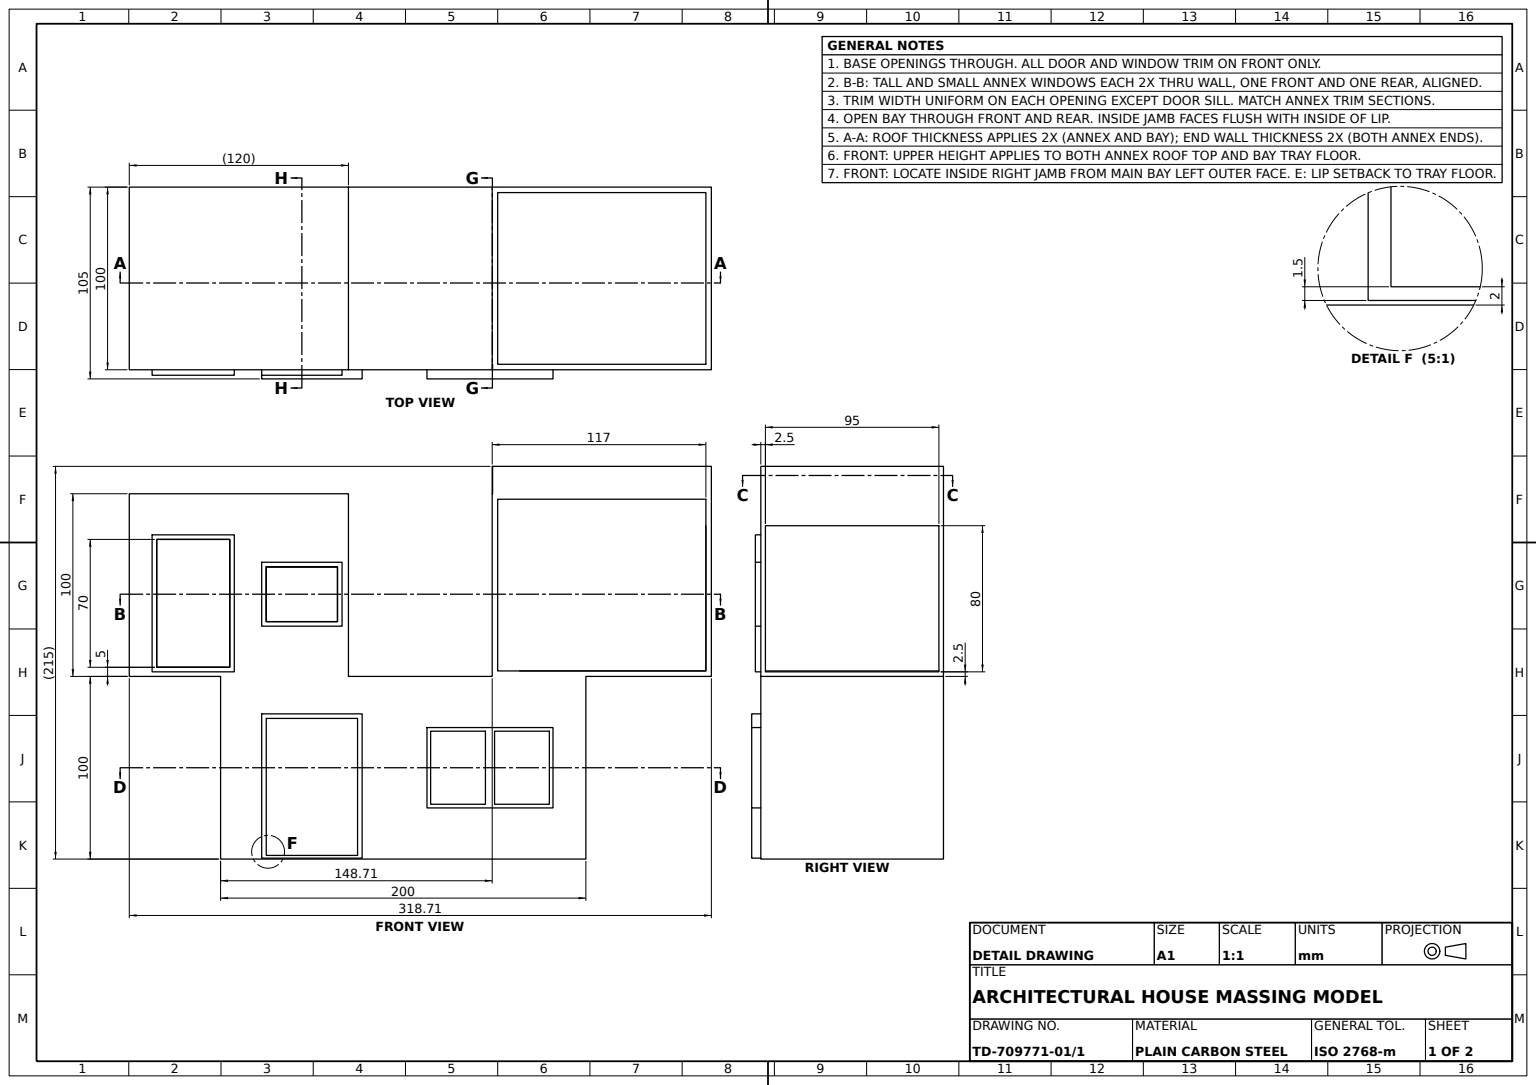
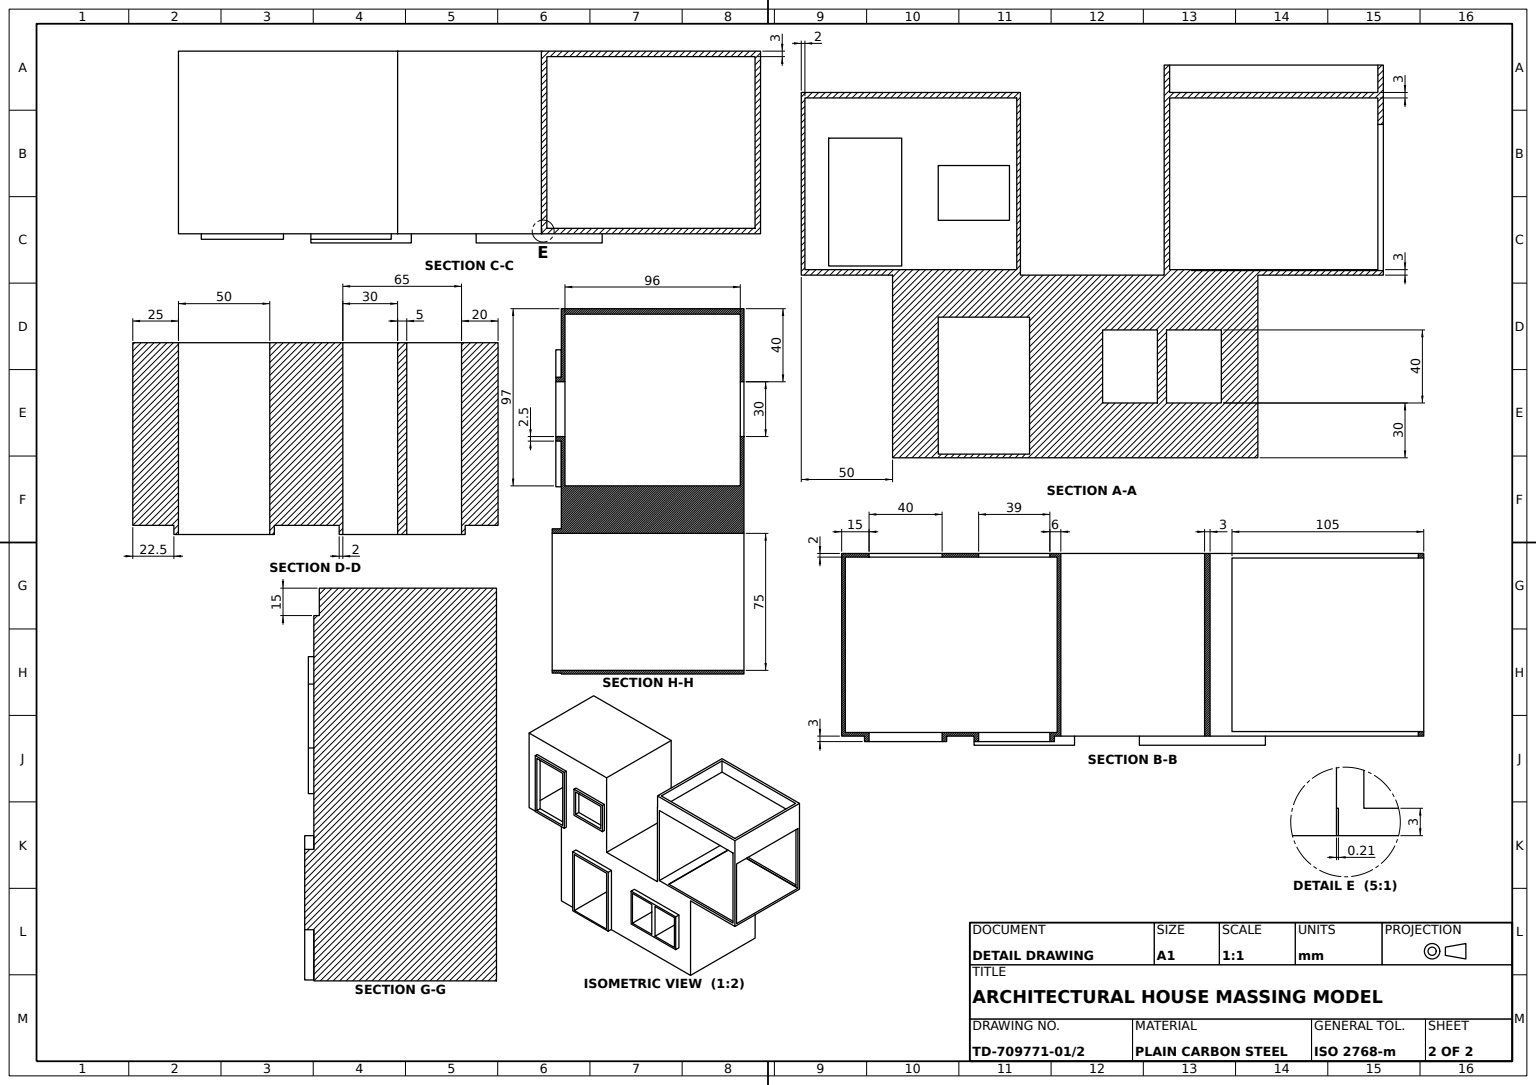
solid
v1 (151.708455,197,-100)
v2 (151.708455,197,0)
e1 v1 v2 LINE
v3 (151.708455,103,0)
e2 v2 v3 LINE
v4 (151.708455,103,-100)
e3 v4 v3 LINE
e4 v1 v4 LINE
face PLANE(AX(P(151.708455,103,-125),D(-1,0,0),D(0,0,1))) rev [e1 e2 -e3 -e4]
v5 (-35,175,-100)
v6 (-35,105,-100)
e5 v5 v6 LINE
v7 (5,105,-100)
e6 v6 v7 LINE
v8 (5,175,-100)
e7 v7 v8 LINE
e8 v8 v5 LINE
v9 (200,0,-100)
v10 (0,0,-100)
e9 v9 v10 LINE
v11 (0,100,-100)
e10 v11 v10 LINE
v12 (-50,100,-100)
e11 v11 v12 LINE
v13 (-50,200,-100)
e12 v13 v12 LINE
v14 (70,200,-100)
e13 v14 v13 LINE
v15 (70,100,-100)
e14 v14 v15 LINE
v16 (148.708455,100,-100)
e15 v16 v15 LINE
v17 (148.708455,215,-100)
e16 v17 v16 LINE
v18 (268.708455,215,-100)
e17 v17 v18 LINE
v19 (268.708455,100,-100)
e18 v18 v19 LINE
v20 (200,100,-100)
e19 v19 v20 LINE
e20 v20 v9 LINE
v21 (150,30,-100)
v22 (150,70,-100)
e21 v21 v22 LINE
v23 (180,30,-100)
e22 v21 v23 LINE
v24 (180,70,-100)
e23 v23 v24 LINE
e24 v24 v22 LINE
v25 (64,160,-100)
v26 (25,160,-100)
e25 v25 v26 LINE
v27 (25,130,-100)
e26 v26 v27 LINE
v28 (64,130,-100)
e27 v27 v28 LINE
e28 v28 v25 LINE
v29 (265.708455,103,-100)
v30 (265.708455,197,-100)
e29 v29 v30 LINE
e30 v30 v1 LINE
e31 v4 v29 LINE
v31 (145,70,-100)
v32 (145,30,-100)
e32 v31 v32 LINE
v33 (115,70,-100)
e33 v31 v33 LINE
v34 (115,30,-100)
e34 v33 v34 LINE
e35 v34 v32 LINE
v35 (25,2,-100)
v36 (75,2,-100)
e36 v35 v36 LINE
v37 (75,77,-100)
e37 v36 v37 LINE
v38 (25,77,-100)
e38 v37 v38 LINE
e39 v38 v35 LINE
face PLANE(AX(P(0,100,-100),D(0,0,1),D(1,0,0))) rev [e5 e6 e7 e8] [e9 -e10 e11 -e12 -e13 e14 -e15 -e16 e17 e18 e19 e20] [-e21 e22 e23 e24] [e25 e26 e27 e28] [e29 e30 e4 e31] [-e32 e33 e34 e35] [e36 e37 e38 e39]
v39 (7.5,177.5,0)
v40 (-37.5,177.5,0)
e40 v39 v40 LINE
v41 (-37.5,177.5,3)
e41 v41 v40 LINE
v42 (7.5,177.5,3)
e42 v42 v41 LINE
e43 v42 v39 LINE
face PLANE(AX(P(-37.5,177.5,3),D(0,-1,0),D(0,0,-1))) rev [e40 -e41 -e42 e43]
v43 (265.708455,103,-2.5)
v44 (163.708455,103,-2.5)
e44 v43 v44 LINE
v45 (265.708455,182.5,-2.5)
e45 v45 v43 LINE
v46 (268.708455,182.5,-2.5)
e46 v45 v46 LINE
v47 (268.708455,102.5,-2.5)
e47 v46 v47 LINE
v48 (163.708455,102.5,-2.5)
e48 v48 v47 LINE
e49 v44 v48 LINE
face PLANE(AX(P(163.708455,102.5,-2.5),D(0,0,1),D(0,-1,0))) rev [-e44 -e45 e46 e47 -e48 -e49]
v49 (0,0,0)
e50 v10 v49 LINE
v50 (0,100,0)
e51 v50 v49 LINE
e52 v11 v50 LINE
face PLANE(AX(P(0,100,0),D(1,0,0),D(0,0,-1))) rev [e50 -e51 -e52 e10]
v51 (-35,175,3)
v52 (-35,105,3)
e53 v51 v52 LINE
v53 (-35,105,-2)
e54 v53 v52 LINE
v54 (-35,175,-2)
e55 v53 v54 LINE
e56 v54 v51 LINE
face PLANE(AX(P(-35,105,-153),D(-1,0,0),D(0,0,1))) rev [e53 -e54 e55 e56]
v55 (64,130,-98)
e57 v28 v55 LINE
v56 (64,160,-98)
e58 v55 v56 LINE
e59 v25 v56 LINE
face PLANE(AX(P(64,130,-153),D(1,0,0),D(0,0,-1))) rev [e57 e58 -e59 -e28]
v57 (268.708455,102.5,-97.5)
e60 v47 v57 LINE
v58 (163.708455,102.5,-97.5)
e61 v58 v57 LINE
e62 v48 v58 LINE
face PLANE(AX(P(163.708455,102.5,-97.5),D(0,-1,0),D(0,0,-1))) rev [e48 e60 -e61 -e62]
v59 (64,160,3)
v60 (25,160,3)
e63 v59 v60 LINE
v61 (64,130,3)
e64 v61 v59 LINE
v62 (25,130,3)
e65 v62 v61 LINE
e66 v60 v62 LINE
v63 (66.5,162.5,3)
v64 (22.5,162.5,3)
e67 v63 v64 LINE
v65 (22.5,127.5,3)
e68 v64 v65 LINE
v66 (66.5,127.5,3)
e69 v65 v66 LINE
e70 v66 v63 LINE
face PLANE(AX(P(0,0,3),D(0,0,-1),D(-1,0,0))) rev [-e63 -e64 -e65 -e66] [e67 e68 e69 e70]
v67 (70,200,0)
e71 v67 v14 LINE
v68 (70,100,0)
e72 v67 v68 LINE
e73 v68 v15 LINE
face PLANE(AX(P(70,200,0),D(-1,0,0),D(0,0,1))) rev [-e14 -e71 e72 e73]
v69 (7.5,102.5,3)
v70 (7.5,102.5,0)
e74 v69 v70 LINE
e75 v70 v39 LINE
e76 v69 v42 LINE
face PLANE(AX(P(7.5,102.5,3),D(-1,0,0),D(0,0,1))) rev [e74 e75 -e43 -e76]
v71 (-48,197,-98)
v72 (-48,197,-2)
e77 v71 v72 LINE
v73 (68,197,-98)
e78 v73 v71 LINE
v74 (68,197,-2)
e79 v74 v73 LINE
e80 v72 v74 LINE
face PLANE(AX(P(0,197,0),D(0,-1,0),D(0,0,-1))) [-e77 -e78 -e79 -e80]
v75 (5,175,-98)
e81 v8 v75 LINE
v76 (-35,175,-98)
e82 v75 v76 LINE
e83 v5 v76 LINE
face PLANE(AX(P(-35,175,-153),D(0,1,0),D(0,0,1))) rev [e81 e82 -e83 -e8]
v77 (163.708455,103,-97.5)
e84 v77 v44 LINE
e85 v58 v77 LINE
face PLANE(AX(P(163.708455,0,0),D(1,0,0),D(0,0,-1))) [e84 e49 e62 e85]
v78 (-35,105,-98)
e86 v76 v78 LINE
e87 v6 v78 LINE
face PLANE(AX(P(-35,105,-153),D(-1,0,0),D(0,0,1))) rev [e86 -e87 -e5 e83]
v79 (-50,200,0)
e88 v13 v79 LINE
e89 v79 v67 LINE
face PLANE(AX(P(0,200,0),D(0,-1,0),D(0,0,-1))) rev [e13 e88 e89 e71]
v80 (113,28,5)
v81 (113,28,0)
e90 v80 v81 LINE
v82 (113,72,5)
e91 v82 v80 LINE
v83 (113,72,0)
e92 v82 v83 LINE
e93 v83 v81 LINE
face PLANE(AX(P(113,72,5),D(1,0,0),D(0,0,-1))) rev [-e90 -e91 e92 e93]
v84 (25,160,-98)
e94 v26 v84 LINE
v85 (25,130,-98)
e95 v84 v85 LINE
e96 v27 v85 LINE
face PLANE(AX(P(25,130,-153),D(-1,0,0),D(0,0,1))) rev [-e26 e94 e95 -e96]
v86 (-50,100,0)
e97 v12 v86 LINE
e98 v79 v86 LINE
face PLANE(AX(P(-50,200,0),D(1,0,0),D(0,0,-1))) rev [e12 e97 -e98 -e88]
v87 (265.708455,215,-97)
v88 (265.708455,215,-3)
e99 v87 v88 LINE
v89 (265.708455,200,-97)
e100 v87 v89 LINE
v90 (265.708455,200,-3)
e101 v90 v89 LINE
e102 v90 v88 LINE
face PLANE(AX(P(265.708455,0,0),D(-1,0,0),D(0,0,1))) [-e99 e100 -e101 e102]
v91 (-37.5,102.5,3)
e103 v41 v91 LINE
e104 v91 v69 LINE
v92 (5,105,3)
e105 v52 v92 LINE
v93 (5,175,3)
e106 v93 v51 LINE
e107 v92 v93 LINE
face PLANE(AX(P(0,0,3),D(0,0,-1),D(-1,0,0))) rev [e42 e103 e104 e76] [-e105 -e53 -e106 -e107]
v94 (5,105,-98)
e108 v94 v75 LINE
e109 v7 v94 LINE
face PLANE(AX(P(5,105,-153),D(1,0,0),D(0,0,-1))) rev [e108 -e81 -e7 e109]
v95 (-37.5,102.5,0)
e110 v40 v95 LINE
e111 v91 v95 LINE
face PLANE(AX(P(-37.5,102.5,3),D(1,0,0),D(0,0,-1))) rev [e41 e110 -e111 -e103]
v96 (64,130,-2)
v97 (25,130,-2)
e112 v96 v97 LINE
v98 (64,160,-2)
e113 v98 v96 LINE
v99 (25,160,-2)
e114 v99 v98 LINE
e115 v97 v99 LINE
v100 (5,105,-2)
e116 v100 v53 LINE
v101 (5,175,-2)
e117 v101 v100 LINE
e118 v54 v101 LINE
v102 (-48,103,-2)
v103 (68,103,-2)
e119 v102 v103 LINE
e120 v102 v72 LINE
e121 v103 v74 LINE
face PLANE(AX(P(-48,103,-2),D(0,0,1),D(1,0,0))) rev [-e112 -e113 -e114 -e115] [-e116 -e117 -e118 -e55] [-e119 e120 e80 -e121]
v104 (25,2,5)
e122 v35 v104 LINE
v105 (25,77,5)
e123 v38 v105 LINE
e124 v105 v104 LINE
face PLANE(AX(P(25,2,-100),D(-1,0,0),D(0,0,1))) rev [-e122 -e39 e123 e124]
v106 (180,70,5)
v107 (150,70,5)
e125 v106 v107 LINE
v108 (180,30,5)
e126 v108 v106 LINE
v109 (150,30,5)
e127 v109 v108 LINE
e128 v107 v109 LINE
v110 (145,70,5)
v111 (115,70,5)
e129 v110 v111 LINE
v112 (145,30,5)
e130 v112 v110 LINE
v113 (115,30,5)
e131 v113 v112 LINE
e132 v111 v113 LINE
v114 (182,72,5)
e133 v114 v82 LINE
v115 (182,28,5)
e134 v80 v115 LINE
e135 v115 v114 LINE
face PLANE(AX(P(0,0,5),D(0,0,1),D(1,0,0))) [-e125 -e126 -e127 -e128] [-e129 -e130 -e131 -e132] [e133 e91 e134 e135]
v116 (66.5,162.5,0)
e136 v63 v116 LINE
v117 (66.5,127.5,0)
e137 v66 v117 LINE
e138 v117 v116 LINE
face PLANE(AX(P(66.5,127.5,3),D(-1,0,0),D(0,0,1))) rev [-e136 -e70 e137 e138]
e139 v32 v112 LINE
e140 v31 v110 LINE
face PLANE(AX(P(145,70,-100),D(-1,0,0),D(0,0,1))) [e32 e139 e130 -e140]
v118 (22.5,162.5,0)
e141 v116 v118 LINE
e142 v64 v118 LINE
face PLANE(AX(P(22.5,162.5,3),D(0,-1,0),D(0,0,-1))) rev [e141 -e142 -e67 e136]
v119 (151.708455,215,-97)
e143 v119 v87 LINE
v120 (151.708455,200,-97)
e144 v120 v119 LINE
e145 v89 v120 LINE
face PLANE(AX(P(0,0,-97),D(0,0,1),D(1,0,0))) [-e143 -e144 -e145 -e100]
v121 (182,28,0)
e146 v115 v121 LINE
v122 (182,72,0)
e147 v121 v122 LINE
e148 v114 v122 LINE
face PLANE(AX(P(182,72,5),D(-1,0,0),D(0,0,1))) rev [-e135 e146 e147 -e148]
v123 (265.708455,197,0)
e149 v30 v123 LINE
e150 v123 v2 LINE
face PLANE(AX(P(265.708455,197,-125),D(0,1,0),D(-1,0,0))) rev [e149 e150 -e1 -e30]
e151 v97 v62 LINE
e152 v96 v61 LINE
face PLANE(AX(P(25,130,-153),D(0,-1,0),D(0,0,-1))) rev [e151 e65 -e152 e112]
v124 (151.708455,200,-3)
v125 (151.708455,215,-3)
e153 v124 v125 LINE
e154 v120 v124 LINE
e155 v125 v119 LINE
face PLANE(AX(P(151.708455,0,0),D(-1,0,0),D(0,0,1))) rev [-e153 -e154 e144 -e155]
v126 (68,103,-98)
v127 (-48,103,-98)
e156 v126 v127 LINE
e157 v127 v102 LINE
e158 v103 v126 LINE
face PLANE(AX(P(0,103,0),D(0,-1,0),D(0,0,-1))) rev [e156 e157 e119 e158]
v128 (22.5,79.5,0)
v129 (22.5,0.5,0)
e159 v128 v129 LINE
v130 (22.5,0.5,5)
e160 v130 v129 LINE
v131 (22.5,79.5,5)
e161 v131 v130 LINE
e162 v131 v128 LINE
face PLANE(AX(P(22.5,0.5,5),D(1,0,0),D(0,0,-1))) rev [e159 -e160 -e161 e162]
e163 v34 v113 LINE
face PLANE(AX(P(115,30,-100),D(0,-1,0),D(0,0,-1))) rev [e163 e131 -e139 -e35]
v132 (22.5,127.5,0)
e164 v65 v132 LINE
e165 v132 v117 LINE
face PLANE(AX(P(22.5,127.5,3),D(0,1,0),D(0,0,1))) rev [-e69 e164 e165 -e137]
v133 (200,0,0)
e166 v133 v9 LINE
e167 v49 v133 LINE
face PLANE(AX(P(0,0,0),D(0,-1,0),D(0,0,-1))) [-e9 -e166 -e167 -e50]
e168 v124 v90 LINE
face PLANE(AX(P(0,200,0),D(0,1,0),D(0,0,1))) [e145 e154 e168 e101]
e169 v21 v109 LINE
e170 v22 v107 LINE
face PLANE(AX(P(150,70,-100),D(1,0,0),D(0,0,-1))) [e128 -e169 e21 e170]
v134 (268.708455,182.5,-97.5)
e171 v57 v134 LINE
e172 v134 v46 LINE
v135 (268.708455,215,0)
e173 v18 v135 LINE
v136 (268.708455,100,0)
e174 v135 v136 LINE
e175 v136 v19 LINE
face PLANE(AX(P(268.708455,200,-100),D(-1,0,0),D(0,0,1))) rev [-e171 -e60 -e47 -e172] [-e18 e173 e174 e175]
e176 v122 v83 LINE
face PLANE(AX(P(113,72,5),D(0,-1,0),D(0,0,-1))) rev [e148 e176 -e92 -e133]
e177 v33 v111 LINE
face PLANE(AX(P(115,70,-100),D(-1,0,0),D(0,-1,0))) rev [e132 -e163 -e34 e177]
e178 v95 v70 LINE
face PLANE(AX(P(-37.5,102.5,3),D(0,1,0),D(0,0,1))) rev [-e104 e111 e178 -e74]
v137 (200,100,0)
e179 v137 v20 LINE
e180 v137 v136 LINE
face PLANE(AX(P(0,100,0),D(0,1,0),D(0,0,1))) rev [e179 -e19 -e175 -e180]
e181 v88 v125 LINE
face PLANE(AX(P(0,0,-3),D(0,0,1),D(1,0,0))) rev [-e181 -e102 -e168 e153]
v138 (265.708455,182.5,-97.5)
e182 v138 v45 LINE
e183 v138 v134 LINE
face PLANE(AX(P(163.708455,182.5,-97.5),D(0,1,0),D(0,0,1))) rev [e172 -e46 -e182 e183]
e184 v101 v93 LINE
face PLANE(AX(P(-35,175,-153),D(0,1,0),D(0,0,1))) rev [-e56 e118 e184 e106]
e185 v99 v60 LINE
e186 v98 v59 LINE
face PLANE(AX(P(25,160,-153),D(0,1,0),D(0,0,1))) rev [-e185 e114 e186 e63]
v139 (75,2,5)
e187 v36 v139 LINE
v140 (75,77,5)
e188 v139 v140 LINE
e189 v37 v140 LINE
face PLANE(AX(P(75,2,-100),D(1,0,0),D(0,0,-1))) rev [e187 e188 -e189 -e37]
e190 v23 v108 LINE
face PLANE(AX(P(115,30,-100),D(0,-1,0),D(0,0,-1))) rev [e127 -e190 -e22 e169]
e191 v24 v106 LINE
face PLANE(AX(P(180,70,-100),D(1,0,0),D(0,0,-1))) rev [-e191 -e23 e190 e126]
v141 (148.920906,200,-3)
v142 (148.920906,200,0)
e192 v141 v142 LINE
v143 (148.920906,215,0)
e193 v143 v142 LINE
v144 (148.920906,215,-3)
e194 v144 v143 LINE
e195 v144 v141 LINE
face PLANE(AX(P(148.920906,200,-3),D(-1,0,0),D(0,0,1))) [e192 -e193 -e194 e195]
v145 (77.5,0.5,0)
v146 (77.5,79.5,0)
e196 v145 v146 LINE
v147 (77.5,79.5,5)
e197 v147 v146 LINE
v148 (77.5,0.5,5)
e198 v148 v147 LINE
e199 v148 v145 LINE
face PLANE(AX(P(77.5,0.5,5),D(-1,0,0),D(0,0,1))) rev [e196 -e197 -e198 e199]
e200 v85 v55 LINE
face PLANE(AX(P(25,130,-153),D(0,-1,0),D(0,0,-1))) rev [e96 e200 -e57 -e27]
e201 v137 v133 LINE
face PLANE(AX(P(200,100,0),D(-1,0,0),D(0,0,1))) rev [e166 -e20 -e179 e201]
e202 v147 v131 LINE
e203 v146 v128 LINE
face PLANE(AX(P(22.5,79.5,5),D(0,-1,0),D(0,0,-1))) rev [-e162 -e202 e197 e203]
e204 v86 v50 LINE
face PLANE(AX(P(0,100,0),D(0,-1,0),D(0,0,-1))) [-e204 -e97 -e11 e52]
e205 v100 v92 LINE
face PLANE(AX(P(-35,105,-153),D(0,-1,0),D(0,0,-1))) rev [-e205 e116 e54 e105]
e206 v56 v84 LINE
face PLANE(AX(P(25,160,-153),D(0,1,0),D(0,0,1))) rev [e206 -e94 -e25 e59]
e207 v78 v94 LINE
face PLANE(AX(P(-35,105,-153),D(0,-1,0),D(0,0,-1))) rev [e207 -e109 -e6 e87]
e208 v126 v73 LINE
e209 v127 v71 LINE
face PLANE(AX(P(-48,103,-98),D(0,0,-1),D(-1,0,0))) rev [-e156 e208 e78 -e209] [-e95 -e206 -e58 -e200] [-e207 -e86 -e82 -e108]
face PLANE(AX(P(-48,103,-2),D(-1,0,0),D(0,0,1))) rev [-e157 e209 e77 -e120]
face PLANE(AX(P(64,130,-153),D(1,0,0),D(0,0,-1))) rev [e152 e64 -e186 e113]
face PLANE(AX(P(25,130,-153),D(-1,0,0),D(0,0,1))) rev [e185 e66 -e151 e115]
e210 v143 v135 LINE
v149 (148.708455,200,0)
e211 v149 v142 LINE
v150 (148.708455,100,0)
e212 v149 v150 LINE
e213 v68 v150 LINE
v151 (265.708455,103,0)
e214 v3 v151 LINE
e215 v151 v123 LINE
e216 v129 v145 LINE
e217 v118 v132 LINE
e218 v81 v121 LINE
face PLANE(AX(P(0,100,0),D(0,0,-1),D(-1,0,0))) rev [-e210 e193 -e211 e212 -e213 -e72 -e89 e98 e204 e51 e167 -e201 e180 -e174] [-e214 -e2 -e150 -e215] [-e216 -e159 -e203 -e196] [-e138 -e165 -e217 -e141] [-e147 -e218 -e93 -e176] [-e178 -e110 -e40 -e75]
e219 v43 v151 LINE
v152 (265.708455,103,-97.5)
e220 v29 v152 LINE
e221 v152 v138 LINE
face PLANE(AX(P(265.708455,103,-125),D(1,0,0),D(0,0,-1))) rev [e219 e215 -e149 -e29 e220 e221 e182 e45]
v153 (148.708455,200,-3)
e222 v141 v153 LINE
v154 (148.708455,215,-3)
e223 v144 v154 LINE
e224 v153 v154 LINE
face PLANE(AX(P(151.708455,200,-3),D(0,0,1),D(1,0,0))) [-e222 -e195 e223 -e224]
face PLANE(AX(P(115,70,-100),D(0,1,0),D(0,0,1))) rev [-e170 -e24 e191 e125]
e225 v140 v105 LINE
e226 v104 v139 LINE
e227 v130 v148 LINE
face PLANE(AX(P(0,0,5),D(0,0,-1),D(-1,0,0))) rev [-e225 -e188 -e226 -e124] [e198 e202 e161 e227]
e228 v154 v17 LINE
face PLANE(AX(P(265.708455,215,0),D(0,1,0),D(0,0,1))) [e99 e181 e155 e143] [-e173 -e17 -e228 -e223 e194 e210]
e229 v77 v152 LINE
face PLANE(AX(P(265.708455,103,-125),D(0,-1,0),D(1,0,0))) rev [-e84 e229 -e220 -e31 e3 e214 -e219 e44]
face PLANE(AX(P(163.708455,102.5,-97.5),D(0,0,-1),D(-1,0,0))) rev [e171 -e183 -e221 -e229 -e85 e61]
face PLANE(AX(P(115,70,-100),D(0,1,0),D(0,0,1))) rev [-e177 -e33 e140 e129]
face PLANE(AX(P(113,28,5),D(0,1,0),D(0,0,1))) rev [-e146 -e134 e90 e218]
face PLANE(AX(P(25,77,-100),D(0,1,0),D(0,0,1))) rev [-e123 -e38 e189 e225]
face PLANE(AX(P(25,2,-100),D(0,-1,0),D(0,0,-1))) rev [-e36 e122 e226 -e187]
face PLANE(AX(P(22.5,0.5,5),D(0,1,0),D(0,0,1))) rev [-e227 e160 e216 -e199]
face PLANE(AX(P(5,105,-153),D(1,0,0),D(0,0,-1))) rev [e205 e107 -e184 e117]
face PLANE(AX(P(22.5,127.5,3),D(1,0,0),D(0,0,-1))) rev [e142 e217 -e164 -e68]
e230 v153 v149 LINE
face PLANE(AX(P(0,200,0),D(0,1,0),D(0,0,1))) [e222 e230 e211 -e192]
e231 v16 v150 LINE
face PLANE(AX(P(0,100,0),D(0,-1,0),D(0,0,-1))) rev [e213 -e231 e15 -e73]
face PLANE(AX(P(68,103,-2),D(1,0,0),D(0,0,-1))) rev [-e158 e121 e79 -e208]
face PLANE(AX(P(148.708455,200,-100),D(1,0,0),D(0,0,-1))) rev [e231 -e212 -e230 e224 e228 e16]
